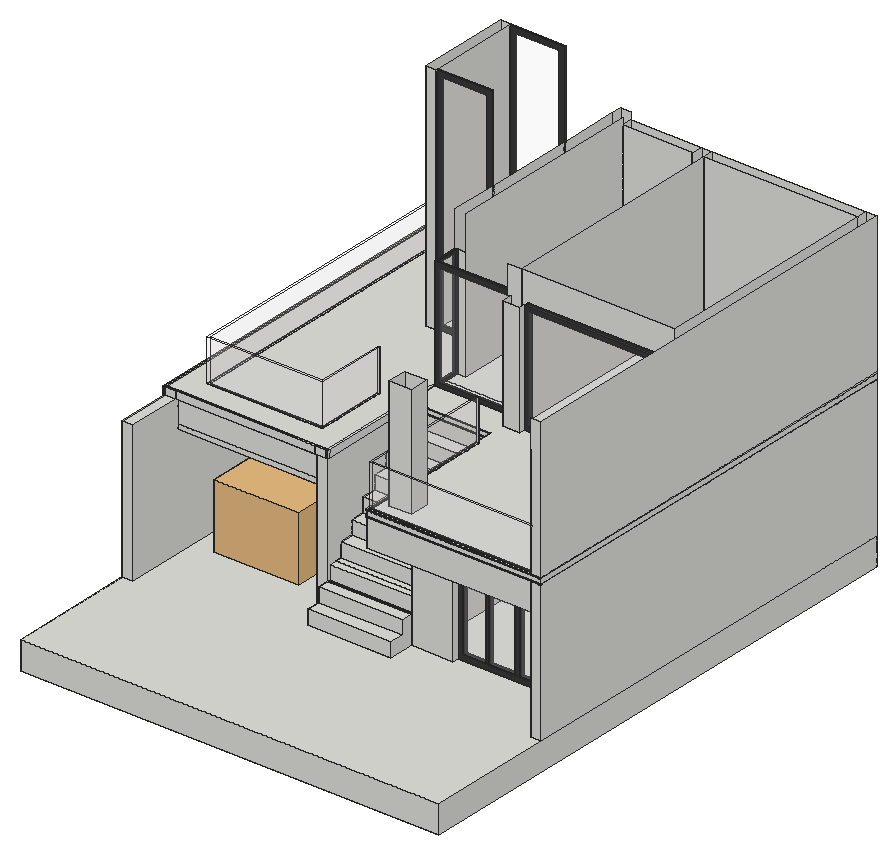
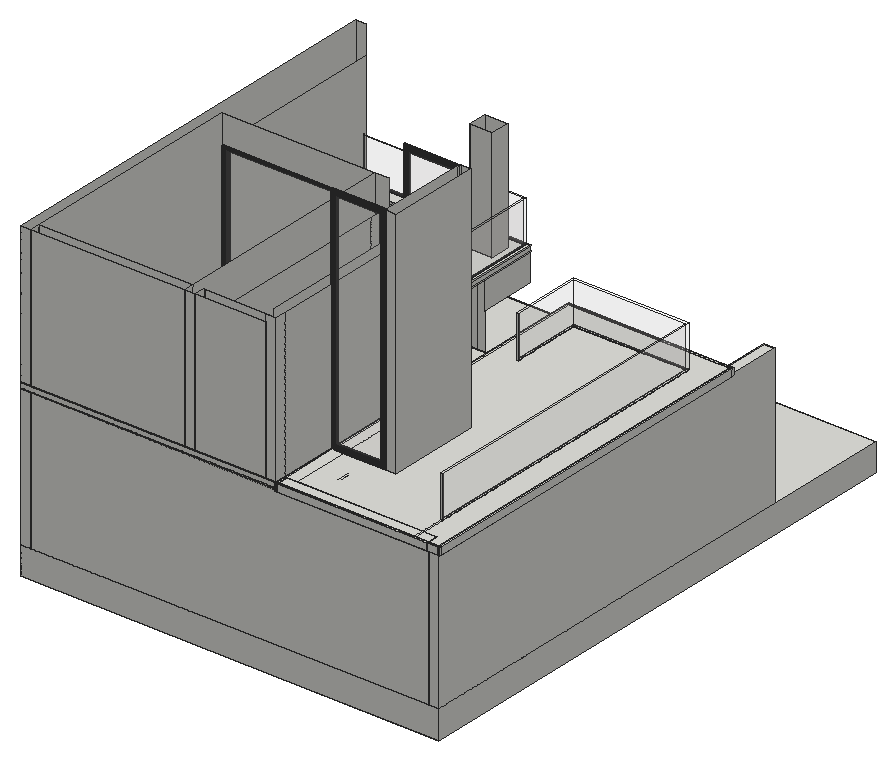
# SketchUp Ruby script. Lengths in inches.
U = 1.inch
M = Sketchup.active_model
def pt(a) = Geom::Point3d.new(a.map { |v| v * U })
def face(e, loops, mat)
  f = e.add_face(loops[0].map { |a| pt(a) })
  loops[1..].each { |l| e.add_face(l.map { |a| pt(a) }).erase! }
  f.material = f.back_material = mat if mat
  f
end
# faces: each face lists its corners as indices into pts; further lists are holes
def faces(e, pts, list, mat = nil) = list.each { |f| face(e, (f[0].is_a?(Array) ? f : [f]).map { |l| l.map { |i| pts[i] } }, mat) }
# xy, xz, yz: faces in a plane at the given z, y or x. An outline is a flat list of corners, or four numbers for a rectangle; further outlines are holes
def ring(l) = l.size == 4 ? [[l[0], l[1]], [l[2], l[1]], [l[2], l[3]], [l[0], l[3]]] : l.each_slice(2).to_a
def flat(e, list, mat, &to3) = list.each { |f| face(e, (f[0].is_a?(Array) ? f : [f]).map { |l| ring(l).map { |u, v| to3.(u, v) } }, mat) }
def xy(e, z, list, mat = nil) = flat(e, list, mat) { |x, y| [x, y, z] }
def xz(e, y, list, mat = nil) = flat(e, list, mat) { |x, z| [x, y, z] }
def yz(e, x, list, mat = nil) = flat(e, list, mat) { |y, z| [x, y, z] }
def lines(e, pts, list) = list.each { |a, b| e.add_line(pt(pts[a]), pt(pts[b])) }
# prism: a flat outline (further loops are holes) pulled along v
def prism(e, loops, v, mat = nil)
  f = face(e, loops, mat); d = Geom::Vector3d.new(v.map { |x| x * U })
  f.pushpull(f.normal.samedirection?(d) ? d.length : -d.length)
end
def box(e, o, s, mat = nil) = prism(e, [[o, [o[0] + s[0], o[1], o[2]], [o[0] + s[0], o[1] + s[1], o[2]], [o[0], o[1] + s[1], o[2]]]], [0, 0, s[2]], mat)
def at(x, y, z, deg = 0) = Geom::Transformation.translation(pt([x, y, z])) * Geom::Transformation.rotation(ORIGIN, Z_AXIS, deg.degrees)
def axes(o, x, y, z) = Geom::Transformation.new([*x, 0, *y, 0, *z, 0, *pt(o).to_a, 1])
def part(name) = M.definitions.add(name)
# library, detail: a bought-in or finely detailed component or shape, given as its bounding box
def library(name, o, s) = part(name).tap { |d| box(d.entities, o, s) }
def detail(e, o, s) = box(e.add_group.entities, o, s)
def put(e, d, t, mat = nil) = e.add_instance(d, t).tap { |i| i.material = mat if mat }
def group(e, t, mat = nil) = e.add_group.tap { |g| g.transformation = t; g.material = mat if mat }.entities
root = M.entities
M.materials.add("Glass Thin Clear 001").color = [255, 250, 250]
M.materials["Glass Thin Clear 001"].alpha = 0.1
M.materials.add("[Color M07]").color = [58, 58, 58]
c1 = library("2016+Honda+Civic+LX+Sedan",[0.01,0.03,0.02],[16.17,34.46,10.62])
xy(root,-24,[[2,0,362,469.5625]])
xy(root,0,[[2,0,362,0,362,109.5625,353,109.5625,353,157.5625,347,157.5625,347,162.0625,248,162.0625,248,157.5625,212,157.5625,212,135.875,140,135.875,140,157.5625,131,157.5625,131,460.5625,11,460.5625,11,109.5625,2,109.5625],[2,109.5625,11,469.5625],[353,109.5625,362,469.5625],[140,135.875,212,135.875,212,157.5625,248,157.5625,248,162.0625,347,162.0625,347,166.5625,221,166.5625,221,460.5625,131,460.5625,131,157.5625,140,157.5625],[140,135.875,212,157.5625],
  [131,157.5625,140,460.5625],[140,157.5625,212,166.5625],[212,157.5625,248,166.5625],[347,157.5625,353,166.5625],[248,162.0625,347,164.5],
  [248,164.5,347,166.3125],[248,166.3125,347,166.5625],[140,166.5625,212,255.875],[212,166.5625,221,460.5625],[221,166.5625,353,460.5625],
  [140,255.875,212,460.5625],[11,460.5625,353,469.5625]])
xy(root,4.7,[[272.2,162.0625,275.1,166.3125],[297.5,162.0625,301.43,166.3125],[322.43,162.0625,325.23,166.3125]])
xy(root,4.7,[[252.7,162.0625,272.2,163.0625],[275.1,162.0625,297.5,163.0625],[301.43,162.0625,322.43,163.0625],[325.23,162.0625,342.3,163.0625],[252.7,163.0625,272.2,166.3125],
  [275.1,163.0625,297.5,166.3125],[301.43,163.0625,322.43,166.3125],[325.23,163.0625,342.3,166.3125]],"[Color M07]")
xy(root,12,[[140,135.875,212,147.875]])
xy(root,24,[[140,147.875,212,157.5625],[140,157.5625,212,159.875]])
xy(root,36,[[140,159.875,212,166.5625],[140,166.5625,212,171.875]])
xy(root,48,[[140,171.875,212,183.875]])
xy(root,60,[[140,183.875,212,195.875]])
xy(root,72,[[140,195.875,212,207.875]])
xy(root,84,[[140,207.875,212,219.875]])
xy(root,91.3,[[272.2,162.0625,275.1,166.3125],[297.5,162.0625,301.43,166.3125],[322.43,162.0625,325.23,166.3125]])
xy(root,91.3,[[252.7,162.0625,272.2,163.0625],[275.1,162.0625,297.5,163.0625],[301.43,162.0625,322.43,163.0625],[325.23,162.0625,342.3,163.0625],[252.7,163.0625,272.2,166.3125],
  [275.1,163.0625,297.5,166.3125],[301.43,163.0625,322.43,166.3125],[325.23,163.0625,342.3,166.3125]],"[Color M07]")
xy(root,96,[[11,157.5625,131,460.5625],[248,157.5625,347,162.0625],[248,166.3125,347,166.5625],[140,219.875,212,231.875]])
xy(root,96,[[248,162.0625,347,164.5],[248,164.5,347,166.3125]],"[Color M07]")
xy(root,96.25,[[212,109.5625,353,157.5625]])
xy(root,100.1875,[[11,157.5625,131,460.5625]])
xy(root,108,[[140,231.875,212,243.875]])
xy(root,120,[[2,109.5625,11,155.5625],[353,109.5625,362,469.5625],[0,155.5625,2,157.5625],[2,155.5625,11,157.5625],[11,155.5625,131,157.5625],
  [131,155.5625,140,157.5625],[140,155.5625,142,157.5625],[0,157.5625,2,469.5625],[2,157.5625,11,469.5625],[131,157.5625,140,460.5625],
  [140,157.5625,142,243.875],[212,157.5625,221,166.5625],[221,157.5625,353,166.5625],[212,166.5625,221,460.5625],[221,166.5625,353,460.5625],
  [140,243.875,142,255.875],[142,243.875,212,255.875],[140,255.875,142,460.5625],[142,255.875,212,460.5625],[11,460.5625,140,469.5625],
  [140,460.5625,142,469.5625],[142,460.5625,353,469.5625],[0,469.5625,2,471.5625],[2,469.5625,11,471.5625],[11,469.5625,140,471.5625],
  [140,469.5625,142,471.5625]])
xy(root,120.125,[[211.8125,109.375,212,243.875],[212,109.375,362,109.5625],[212,109.5625,362,109.5625,362,469.5625,142,469.5625,142,243.875,212,243.875],[142,243.6875,211.8125,243.875]])
xy(root,121,[[211.8125,109.375,212,243.875],[212,109.375,362,109.5625],[212,109.5625,362,109.5625,362,469.5625,142,469.5625,142,243.875,212,243.875],[142,243.6875,211.8125,243.875]])
xy(root,125,[[211.8125,109.375,212,243.875],[212,109.375,362,109.5625],[212,109.5625,362,109.5625,362,469.5625,142,469.5625,142,243.875,212,243.875],[142,243.6875,211.8125,243.875]])
xy(root,126,[[[211.8125,109.375,353,109.375,353,111.13,213.57,111.13,213.57,226.42,214.91,226.42,214.91,112.47,353,112.47,353,260.1875,226.85,260.1875,226.85,255.6875,211.8125,255.6875,211.8125,269.93,142,269.93,142,243.6875,211.8125,243.6875],[220.8125,122.73,239.9375,139.05]],[353,109.375,362,469.5625],[213.57,111.13,213.57,226.42,214.91,226.42,214.91,112.47,353,112.47,353,111.13],[220.8125,122.73,239.9375,139.05],[0,155.5625,2,157.5625],
  [2,155.5625,11,157.5625],[11,155.5625,131,157.5625],[131,155.5625,140,157.5625],[140,155.5625,142,157.5625],[0,157.5625,2,469.5625],
  [2,157.5625,140,157.5625,140,331.125,95,331.125,95,330.5625,86,330.5625,86,411.125,95,411.125,95,410.9375,131,410.9375,131,460.5625,23.16,460.5625,23.16,178.72,118.84,178.72,118.84,238.125,120.75,238.125,120.75,176.82,21.25,176.82,21.25,460.5625,11,460.5625,11,469.5625,2,469.5625],[140,157.5625,142,331.125],[21.25,176.82,21.25,441.31,23.16,441.31,23.16,178.72,118.84,178.72,118.84,238.125,120.75,238.125,120.75,176.82],[211.8125,255.6875,226.85,264.6875],[226.85,264.4375,353,264.6875],
  [211.8125,264.6875,211.8125,269.93,213.3125,269.93,213.3125,272.05,211.8125,272.05,211.8125,469.5625,220.8125,469.5625,220.8125,264.6875],[220.8125,264.6875,353,460.5625],[143.5,269.93,211.8125,271.43],[143.5,271.43,211.8125,272.05],[144.125,272.05,211.8125,280.43],
  [144.125,280.43,211.8125,280.43,211.8125,460.5625,151,460.5625,151,292.12,144.125,292.12],[142,292.12,151,469.5625],[86,330.5625,95,411.125],[95,332.75,142,333.43],[95,333.43,131,409.3125],
  [131,333.43,140,409.3125],[140,333.43,142,409.3125],[131,410.9375,140,460.5625],[140,410.9375,142,460.5625],[21.25,441.31,23.16,460.5625],
  [11,460.5625,21.25,469.5625],[21.25,460.5625,23.16,469.5625],[23.16,460.5625,140,469.5625],[140,460.5625,142,469.5625],[151,460.5625,211.8125,469.5625],
  [220.8125,460.5625,353,469.5625],[0,469.5625,2,471.5625],[2,469.5625,11,471.5625],[11,469.5625,140,471.5625],[140,469.5625,142,471.5625]])
xy(root,126,[[226.85,260.1875,353,262.625],[226.85,262.625,353,264.4375],[142,269.93,143.5,271.43],[211.8125,269.93,213.3125,271.43],[142,271.43,143.5,272.05],
  [211.8125,271.43,213.3125,272.05],[142,272.05,143.5,280.43],[143.5,272.05,144.125,280.43],[142,280.43,143.5,292.12],[143.5,280.43,144.125,292.12],
  [95,331.125,131,332.125],[131,331.125,140,332.125],[140,331.125,142,332.125],[95,332.125,131,332.75],[131,332.125,140,332.75],
  [140,332.125,142,332.75],[95,409.3125,131,410.3125],[131,409.3125,140,410.3125],[140,409.3125,142,410.3125],[95,410.3125,131,410.9375],
  [131,410.3125,140,410.9375],[140,410.3125,142,410.9375]],"[Color M07]")
xz(root,0,[[2,-24,362,0]])
xz(root,109.375,[[211.8125,120.125,362,121],[211.8125,125,362,126],[353,126,362,126,362,246,353,246,353,163.1875,354.76,163.1875,354.76,162,353,162]])
xz(root,109.5625,[[2,0,11,120],[353,0,362,120],[212,96.25,353,96.25,353,120,362,120,362,120.125,212,120.125],[212,121,362,125]])
xz(root,111.13,[[213.57,126,353,162]],"Glass Thin Clear 001")
xz(root,112.47,[[214.91,126,353,162]],"Glass Thin Clear 001")
xz(root,122.73,[[220.8125,126,239.9375,222]])
xz(root,135.875,[[140,0,212,12]])
xz(root,139.05,[[220.8125,126,239.9375,222]])
xz(root,147.875,[[140,12,212,24]])
xz(root,155.5625,[[0,120,2,126],[2,120,11,126],[11,120,131,126],[131,120,140,126],[140,120,142,126]])
xz(root,157.5625,[[131,0,140,120],[140,0,212,24],[212,0,248,0,248,96,347,96,347,0,353,0,353,96.25,212,96.25],[11,96,131,100.1875],[212,96.25,221,120],
  [221,96.25,353,120],[11,100.1875,131,120],[0,120,2,126],[2,120,11,126],[11,120,131,126],
  [131,120,140,126],[140,120,142,126]])
xz(root,159.875,[[140,24,212,36]])
xz(root,162.0625,[[[248,0,347,96],[252.7,4.7,342.3,91.3]],[272.2,4.7,275.1,91.3],[297.5,4.7,301.43,91.3],[322.43,4.7,325.23,91.3]],"[Color M07]")
xz(root,163.0625,[[252.7,4.7,272.2,91.3],[275.1,4.7,297.5,91.3],[301.43,4.7,322.43,91.3],[325.23,4.7,342.3,91.3]],"Glass Thin Clear 001")
xz(root,164.5,[[248,0,347,96]],"Glass Thin Clear 001")
xz(root,166.3125,[[[248,0,347,96],[252.7,4.7,342.3,91.3]],[272.2,4.7,275.1,91.3],[297.5,4.7,301.43,91.3],[322.43,4.7,325.23,91.3]],"[Color M07]")
xz(root,166.5625,[[140,0,212,36],[212,0,221,120],[221,0,221,120,353,120,353,0,347,0,347,96,248,96,248,0]])
xz(root,171.875,[[140,36,212,48]])
xz(root,176.82,[[21.25,126,120.75,162]],"Glass Thin Clear 001")
xz(root,178.72,[[23.16,126,118.84,162]],"Glass Thin Clear 001")
xz(root,183.875,[[140,48,212,60]])
xz(root,195.875,[[140,60,212,72]])
xz(root,207.875,[[140,72,212,84]])
xz(root,219.875,[[140,84,212,96]])
xz(root,226.42,[[213.57,126,214.91,162]])
xz(root,231.875,[[140,96,212,108]])
xz(root,238.125,[[118.84,126,120.75,162]])
xz(root,243.6875,[[142,120.125,211.8125,121],[142,125,211.8125,126]])
xz(root,243.875,[[140,108,212,120],[142,120,212,120.125],[142,121,212,125]])
xz(root,255.6875,[[211.8125,126,226.85,222]])
xz(root,255.875,[[140,0,212,120]])
xz(root,260.1875,[[[226.85,126,353,222],[230.23,129.38,349.62,218.62]]],"[Color M07]")
xz(root,262.625,[[226.85,126,353,222]],"Glass Thin Clear 001")
xz(root,264.4375,[[[226.85,126,353,222],[230.23,129.38,349.62,218.62]]],"[Color M07]")
xz(root,264.6875,[[211.8125,126,211.8125,222,209.4375,222,209.4375,246,220.8125,246,220.8125,126],[220.8125,126,220.8125,246,353,246,353,222,226.85,222,226.85,126]])
xz(root,269.93,[[[142,126,213.3125,222],[146.125,129.6875,209.625,218.3125]]],"[Color M07]")
xz(root,271.43,[[143.5,126,213.3125,222]],"Glass Thin Clear 001")
xz(root,272.05,[[142,126,144.125,222]])
xz(root,272.05,[[[144.125,126,213.3125,222],[146.125,129.6875,209.625,218.3125]]],"[Color M07]")
xz(root,292.12,[[144.125,126,151,222]])
xz(root,292.12,[[142,126,143.5,222],[143.5,126,144.125,222]],"[Color M07]")
xz(root,330.5625,[[86,126,95,325.875]])
xz(root,331.125,[[[95,126,142,325.875],[99.31,130.31,137.69,321.57]]],"[Color M07]")
xz(root,332.125,[[95,126,142,325.875]],"Glass Thin Clear 001")
xz(root,332.75,[[[95,126,142,325.875],[99.31,130.31,137.69,321.57]]],"[Color M07]")
xz(root,409.3125,[[[95,126,142,325.875],[99.31,130.31,137.69,321.57]]],"[Color M07]")
xz(root,410.3125,[[95,126,142,325.875]],"Glass Thin Clear 001")
xz(root,410.9375,[[[95,126,142,325.875],[99.31,130.31,137.69,321.57]]],"[Color M07]")
xz(root,411.125,[[86,126,95,325.875]])
xz(root,441.31,[[21.25,126,23.16,162]])
xz(root,460.5625,[[11,0,131,96],[131,0,140,120],[140,0,212,120],[212,0,221,120],[221,0,353,120],
  [11,96,131,100.1875],[11,100.1875,131,120],[11,120,131,126],[131,120,140,126],[140,120,142,126],
  [151,126,211.8125,126,211.8125,222,209.4375,222,209.4375,246,151,246],[220.8125,126,353,246]])
xz(root,469.5625,[[2,-24,362,0],[2,0,11,120],[11,0,353,120],[353,0,362,120],[0,120,2,126],
  [2,120,11,126],[11,120,140,126],[140,120,142,126],[142,120,362,120.125],[142,120.125,362,121],
  [142,121,362,125],[142,125,362,126],[142,126,151,252],[151,126,211.8125,246],[211.8125,126,220.8125,246],
  [220.8125,126,353,246],[353,126,362,246]])
xz(root,471.5625,[[0,120,2,126],[2,120,11,126],[11,120,140,126],[140,120,142,126]])
yz(root,0,[[155.5625,120,157.5625,126],[157.5625,120,469.5625,126],[469.5625,120,471.5625,126]])
yz(root,2,[[0,-24,469.5625,0],[109.5625,0,469.5625,120],[155.5625,120,157.5625,126],[157.5625,120,469.5625,126],[469.5625,120,471.5625,126]])
yz(root,11,[[109.5625,0,460.5625,0,460.5625,96,157.5625,96,157.5625,120,109.5625,120],[460.5625,0,469.5625,120],[157.5625,96,460.5625,100.1875],[157.5625,100.1875,460.5625,120],[155.5625,120,157.5625,126],
  [460.5625,120,469.5625,126],[469.5625,120,471.5625,126]])
yz(root,21.25,[[176.82,126,441.31,162]],"Glass Thin Clear 001")
yz(root,23.16,[[178.72,126,441.31,162]],"Glass Thin Clear 001")
yz(root,86,[[330.5625,126,411.125,325.875]])
yz(root,95,[[330.5625,126,331.125,325.875],[332.75,126,333.43,325.875],[333.43,126,409.3125,325.875],[410.9375,126,411.125,325.875]])
yz(root,95,[[331.125,126,332.125,325.875],[332.125,126,332.75,325.875],[409.3125,126,410.3125,325.875],[410.3125,126,410.9375,325.875]],"[Color M07]")
yz(root,118.84,[[178.72,126,238.125,162]],"Glass Thin Clear 001")
yz(root,120.75,[[176.82,126,238.125,162]],"Glass Thin Clear 001")
yz(root,131,[[157.5625,0,460.5625,96],[157.5625,96,460.5625,100.1875],[157.5625,100.1875,460.5625,120],[155.5625,120,157.5625,126]])
yz(root,140,[[135.875,0,135.875,12,147.875,12,147.875,24,157.5625,24,157.5625,0],[166.5625,0,166.5625,36,171.875,36,171.875,48,183.875,48,183.875,60,195.875,60,195.875,72,207.875,72,207.875,84,219.875,84,219.875,96,231.875,96,231.875,108,243.875,108,243.875,120,255.875,120,255.875,0],[255.875,0,460.5625,120],[157.5625,24,159.875,24,159.875,36,171.875,36,171.875,48,183.875,48,183.875,60,195.875,60,195.875,72,207.875,72,207.875,84,219.875,84,219.875,96,231.875,96,231.875,108,243.875,108,243.875,120,157.5625,120],[155.5625,120,157.5625,126],
  [460.5625,120,469.5625,126],[469.5625,120,471.5625,126]])
yz(root,142,[[155.5625,120,157.5625,126],[157.5625,120,243.875,120,243.875,120.125,243.6875,120.125,243.6875,121,243.875,121,243.875,125,243.6875,125,243.6875,126,157.5625,126],[243.875,120,460.5625,120.125],[460.5625,120,469.5625,120.125],[469.5625,120,471.5625,126],
  [243.6875,120.125,460.5625,121],[460.5625,120.125,469.5625,121],[243.875,121,460.5625,125],[460.5625,121,469.5625,125],[243.6875,125,460.5625,126],
  [460.5625,125,469.5625,126],[292.12,126,331.125,252],[332.75,126,333.43,252],[333.43,126,409.3125,252],[410.9375,126,460.5625,252],
  [460.5625,126,469.5625,252]])
yz(root,142,[[269.93,126,272.05,222],[[272.05,126,292.12,222],[272.42,128.05,290.07,219.95]],[331.125,126,332.125,252],[332.125,126,332.75,252],[409.3125,126,410.3125,252],
  [410.3125,126,410.9375,252]],"[Color M07]")
yz(root,143.5,[[270.37,126,271.43,222]])
yz(root,143.5,[[271.43,126,292.12,222]],"Glass Thin Clear 001")
yz(root,144.125,[[[272.05,126,292.12,222],[272.42,128.05,290.07,219.95]]],"[Color M07]")
yz(root,151,[[292.12,126,460.5625,252],[460.5625,126,469.5625,246]])
yz(root,211.8125,[[109.375,120.125,243.6875,121],[109.375,125,243.6875,126],[255.6875,126,264.6875,222],[264.6875,126,280.43,222],[280.43,126,460.5625,222],
  [460.5625,126,469.5625,246]])
yz(root,212,[[135.875,0,157.5625,0,157.5625,24,147.875,24,147.875,12,135.875,12],[157.5625,0,166.5625,0,166.5625,36,159.875,36,159.875,24,157.5625,24],[166.5625,0,255.875,0,255.875,120,243.875,120,243.875,108,231.875,108,231.875,96,219.875,96,219.875,84,207.875,84,207.875,72,195.875,72,195.875,60,183.875,60,183.875,48,171.875,48,171.875,36,166.5625,36],[255.875,0,460.5625,120],[157.5625,24,157.5625,120,166.5625,120,166.5625,36,159.875,36,159.875,24],
  [166.5625,36,166.5625,120,243.875,120,243.875,108,231.875,108,231.875,96,219.875,96,219.875,84,207.875,84,207.875,72,195.875,72,195.875,60,183.875,60,183.875,48,171.875,48,171.875,36],[109.5625,96.25,109.5625,120.125,243.875,120.125,243.875,120,157.5625,120,157.5625,96.25],[109.5625,121,243.875,125]])
yz(root,213.3125,[[269.93,126,271.43,222],[271.43,126,272.05,222]],"[Color M07]")
yz(root,213.57,[[111.13,126,226.42,162]],"Glass Thin Clear 001")
yz(root,214.91,[[112.47,126,226.42,162]],"Glass Thin Clear 001")
yz(root,220.8125,[[122.73,126,139.05,222],[264.6875,126,460.5625,246],[460.5625,126,469.5625,246]])
yz(root,221,[[166.5625,0,460.5625,120]])
yz(root,226.85,[[255.6875,126,260.1875,222],[264.4375,126,264.6875,222]])
yz(root,226.85,[[260.1875,126,262.625,222],[262.625,126,264.4375,222]],"[Color M07]")
yz(root,239.9375,[[122.73,126,139.05,222]])
yz(root,248,[[157.5625,0,162.0625,96],[166.3125,0,166.5625,96]])
yz(root,248,[[162.0625,0,164.5,96],[164.5,0,166.3125,96]],"[Color M07]")
yz(root,252.7,[[162.0625,4.7,163.0625,91.3],[163.0625,4.7,166.3125,91.3]],"[Color M07]")
yz(root,272.2,[[162.0625,4.7,163.0625,91.3],[163.0625,4.7,166.3125,91.3]],"[Color M07]")
yz(root,275.1,[[162.0625,4.7,163.0625,91.3],[163.0625,4.7,166.3125,91.3]],"[Color M07]")
yz(root,297.5,[[162.0625,4.7,163.0625,91.3],[163.0625,4.7,166.3125,91.3]],"[Color M07]")
yz(root,301.43,[[162.0625,4.7,163.0625,91.3],[163.0625,4.7,166.3125,91.3]],"[Color M07]")
yz(root,322.43,[[162.0625,4.7,163.0625,91.3],[163.0625,4.7,166.3125,91.3]],"[Color M07]")
yz(root,325.23,[[162.0625,4.7,163.0625,91.3],[163.0625,4.7,166.3125,91.3]],"[Color M07]")
yz(root,342.3,[[162.0625,4.7,163.0625,91.3],[163.0625,4.7,166.3125,91.3]],"[Color M07]")
yz(root,347,[[157.5625,0,162.0625,96],[166.3125,0,166.5625,96]])
yz(root,347,[[162.0625,0,164.5,96],[164.5,0,166.3125,96]],"[Color M07]")
yz(root,353,[[109.5625,0,157.5625,96.25],[157.5625,0,166.5625,120],[166.5625,0,460.5625,120],[460.5625,0,469.5625,120],[109.5625,96.25,157.5625,120],
  [109.375,126,109.375,222,260.1875,222,260.1875,126,112.47,126,112.47,163.1875,111.13,163.1875,111.13,126],[111.13,126,112.47,162],[264.4375,126,264.6875,222],[264.6875,126,460.5625,246],[460.5625,126,469.5625,246]])
yz(root,353,[[260.1875,126,262.625,222],[262.625,126,264.4375,222]],"[Color M07]")
yz(root,362,[[0,-24,469.5625,0],[109.5625,0,469.5625,120],[109.5625,120,469.5625,120.125],[109.375,120.125,469.5625,121],[109.5625,121,469.5625,125],
  [109.375,125,469.5625,126],[109.375,126,469.5625,246]])
p = [[109.84,432.28,126],[109.84,439.4,126],[111.75,430.38,126],[111.75,441.31,126]]
lines(root,p,[[0,1],[2,3]])
put(root,c1,axes([28.25,174.78,-0.09],[4.5312,0,0],[0,3.3696,0],[0,0,5.23]))
